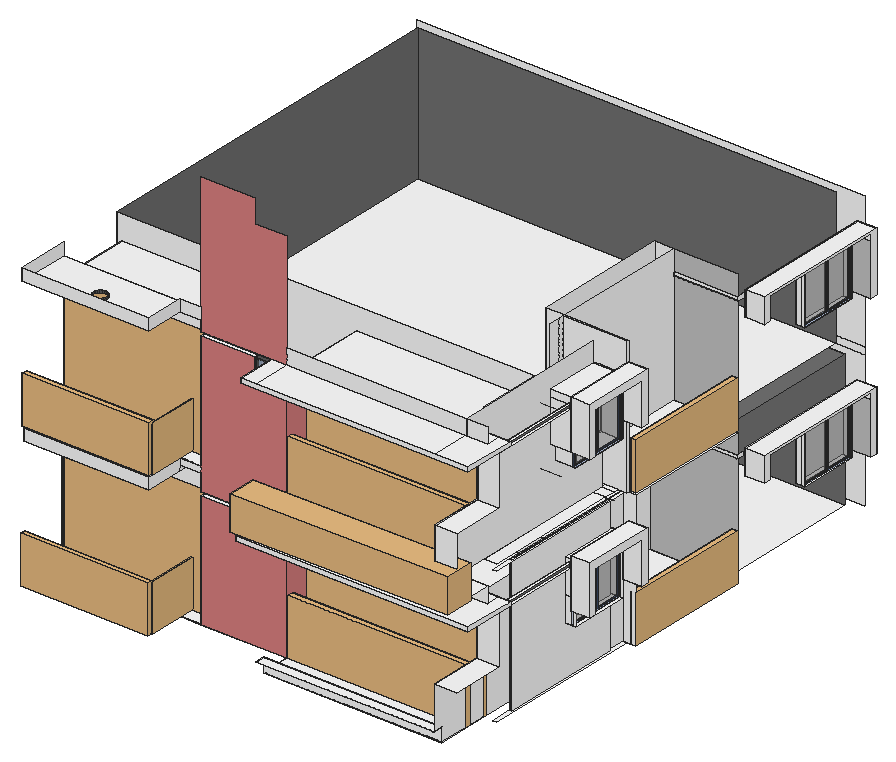
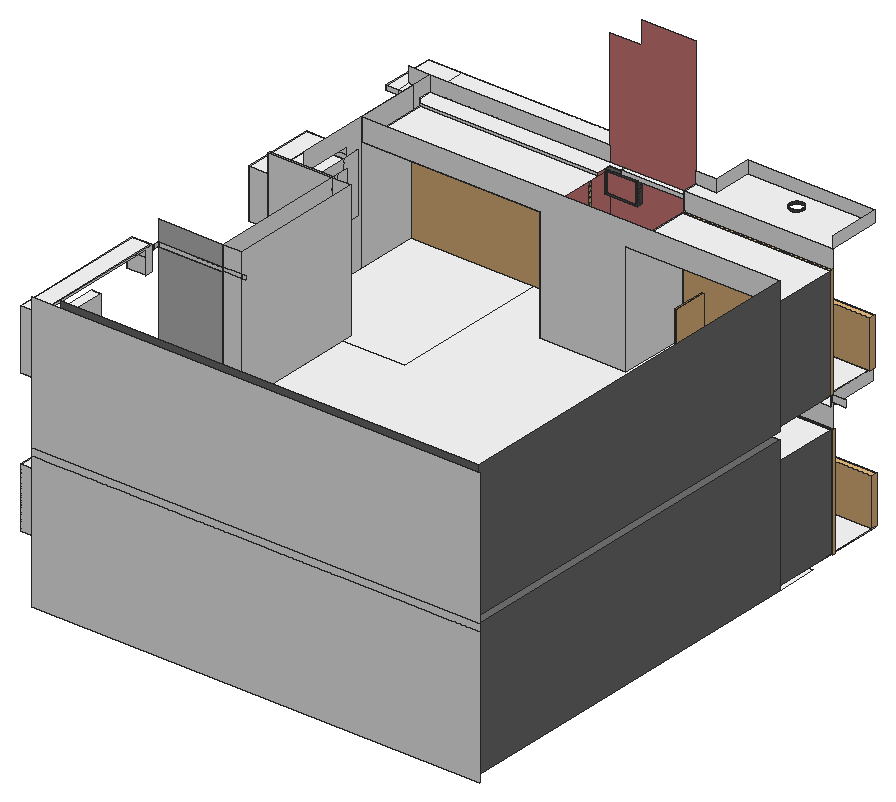
# SketchUp Ruby script. Lengths in inches.
U = 1.inch
M = Sketchup.active_model
def pt(a) = Geom::Point3d.new(a.map { |v| v * U })
def face(e, loops, mat)
  f = e.add_face(loops[0].map { |a| pt(a) })
  loops[1..].each { |l| e.add_face(l.map { |a| pt(a) }).erase! }
  f.material = f.back_material = mat if mat
  f
end
# faces: each face lists its corners as indices into pts; further lists are holes
def faces(e, pts, list, mat = nil) = list.each { |f| face(e, (f[0].is_a?(Array) ? f : [f]).map { |l| l.map { |i| pts[i] } }, mat) }
# xy, xz, yz: faces in a plane at the given z, y or x. An outline is a flat list of corners, or four numbers for a rectangle; further outlines are holes
def ring(l) = l.size == 4 ? [[l[0], l[1]], [l[2], l[1]], [l[2], l[3]], [l[0], l[3]]] : l.each_slice(2).to_a
def flat(e, list, mat, &to3) = list.each { |f| face(e, (f[0].is_a?(Array) ? f : [f]).map { |l| ring(l).map { |u, v| to3.(u, v) } }, mat) }
def xy(e, z, list, mat = nil) = flat(e, list, mat) { |x, y| [x, y, z] }
def xz(e, y, list, mat = nil) = flat(e, list, mat) { |x, z| [x, y, z] }
def yz(e, x, list, mat = nil) = flat(e, list, mat) { |y, z| [x, y, z] }
def lines(e, pts, list) = list.each { |a, b| e.add_line(pt(pts[a]), pt(pts[b])) }
# prism: a flat outline (further loops are holes) pulled along v
def prism(e, loops, v, mat = nil)
  f = face(e, loops, mat); d = Geom::Vector3d.new(v.map { |x| x * U })
  f.pushpull(f.normal.samedirection?(d) ? d.length : -d.length)
end
def box(e, o, s, mat = nil) = prism(e, [[o, [o[0] + s[0], o[1], o[2]], [o[0] + s[0], o[1] + s[1], o[2]], [o[0], o[1] + s[1], o[2]]]], [0, 0, s[2]], mat)
def at(x, y, z, deg = 0) = Geom::Transformation.translation(pt([x, y, z])) * Geom::Transformation.rotation(ORIGIN, Z_AXIS, deg.degrees)
def axes(o, x, y, z) = Geom::Transformation.new([*x, 0, *y, 0, *z, 0, *pt(o).to_a, 1])
def part(name) = M.definitions.add(name)
# library, detail: a bought-in or finely detailed component or shape, given as its bounding box
def library(name, o, s) = part(name).tap { |d| box(d.entities, o, s) }
def detail(e, o, s) = box(e.add_group.entities, o, s)
def put(e, d, t, mat = nil) = e.add_instance(d, t).tap { |i| i.material = mat if mat }
def group(e, t, mat = nil) = e.add_group.tap { |g| g.transformation = t; g.material = mat if mat }.entities
root = M.entities
M.materials.add("[Color M00]").color = [255, 255, 255]
M.materials.add("[Color M02]").color = [198, 198, 198]
M.materials.add("[Color M05]").color = [114, 114, 114]
M.materials.add("[Color M06]").color = [86, 86, 86]
M.materials.add("[Color_006]").color = [86, 86, 86]
M.materials.add("[Tile Various Tan]").color = [221, 130, 130]
M.materials.add("[Translucent Glass Blue]").color = [74, 111, 178]
M.materials["[Translucent Glass Blue]"].alpha = 0.26
M.materials.add("[Translucent Glass Gray]").color = [128, 128, 128]
M.materials["[Translucent Glass Gray]"].alpha = 0.5
M.materials.add("[Translucent_Glass_Gray]").color = [167, 187, 214]
M.materials["[Translucent_Glass_Gray]"].alpha = 0.8
c1 = library("Glazed balcony doors",[0,0,0],[135.86,2.83,115.35])
c2 = library("Glass Railing",[0,0,0],[139.5,4.76,42])
c3 = part("glass-railing")
detail(c3.entities,[0,0,0],[1.26,75.59,33.1875])
c4 = part("Group\#3")
xy(c4.entities,0,[[0,0,32.48,1.97]])
xy(c4.entities,0.98,[[0.98,0,31.5,0.98],[0.98,0.98,31.5,1.97]])
xy(c4.entities,8.86,[[0.98,0,31.5,0.98],[0.98,0.98,31.5,1.97]])
xy(c4.entities,9.84,[[0,0,32.48,1.97]])
xz(c4.entities,0,[[[0,0,32.48,9.84],[0.98,0.98,31.5,8.86]]])
xz(c4.entities,0.98,[[0.98,0.98,31.5,8.86]],"[Translucent Glass Gray]")
xz(c4.entities,1.97,[[[0,0,32.48,9.84],[0.98,0.98,31.5,8.86]]])
yz(c4.entities,0,[[0,0,1.97,9.84]])
yz(c4.entities,0.98,[[0,0.98,0.98,8.86],[0.98,0.98,1.97,8.86]])
yz(c4.entities,31.5,[[0,0.98,0.98,8.86],[0.98,0.98,1.97,8.86]])
yz(c4.entities,32.48,[[0,0,1.97,9.84]])
c5 = part("Group\#4")
xy(c5.entities,0,[[0,0,32.48,1.97]])
xy(c5.entities,0.98,[[0.98,0,31.5,0.98],[0.98,0.98,31.5,1.97]])
xy(c5.entities,71.85,[[0.98,0,31.5,0.98],[0.98,0.98,31.5,1.97]])
xy(c5.entities,72.83,[[0,0,32.48,1.97]])
xz(c5.entities,0,[[[0,0,32.48,72.83],[0.98,0.98,31.5,71.85]]])
xz(c5.entities,0.98,[[0.98,0.98,31.5,71.85]],"[Translucent Glass Gray]")
xz(c5.entities,1.97,[[[0,0,32.48,72.83],[0.98,0.98,31.5,71.85]]])
yz(c5.entities,0,[[0,0,1.97,72.83]])
yz(c5.entities,0.98,[[0,0.98,0.98,71.85],[0.98,0.98,1.97,71.85]])
yz(c5.entities,31.5,[[0,0.98,0.98,71.85],[0.98,0.98,1.97,71.85]])
yz(c5.entities,32.48,[[0,0,1.97,72.83]])
c6 = part("Fixed transom window")
xy(c6.entities,0,[[0,0,70.86,3.9375]])
xy(c6.entities,1.97,[[1.97,0,34.45,0.98],[36.42,0,68.9,3.9375],[1.97,2.95,34.45,3.9375]])
xy(c6.entities,86.61,[[1.97,0,34.45,3.9375],[34.45,0,36.42,3.9375],[36.42,0,68.9,3.9375]])
xy(c6.entities,88.58,[[0,0,70.86,3.9375]])
xz(c6.entities,0,[[[0,0,70.86,88.58],[1.97,1.97,34.45,86.61],[36.42,1.97,68.9,86.61]]])
xz(c6.entities,3.9375,[[[0,0,70.86,88.58],[1.97,1.97,34.45,86.61],[36.42,1.97,68.9,86.61]]])
yz(c6.entities,0,[[0,0,3.9375,88.58]])
yz(c6.entities,1.97,[[0,1.97,3.9375,74.8],[0,76.77,3.9375,86.61]])
yz(c6.entities,34.45,[[0,1.97,3.9375,86.61]])
yz(c6.entities,36.42,[[0,1.97,3.9375,86.61]])
yz(c6.entities,68.9,[[0,1.97,3.9375,86.61]])
yz(c6.entities,70.86,[[0,0,3.9375,88.58]])
g1 = group(c6.entities,at(1.97,0,74.8))
box(g1,[0,0,0],[66.93,3.9375,1.97])
put(c6.entities,c4,at(1.97,0.98,76.77),"[Translucent Glass Blue]")
put(c6.entities,c4,at(36.42,0.98,76.77),"[Translucent Glass Blue]")
put(c6.entities,c5,at(1.97,0.98,1.97),"[Translucent Glass Blue]")
put(c6.entities,c5,at(36.42,0.98,1.97),"[Translucent Glass Blue]")
c7 = part("FIXED+GLASS+WINDOW+WITH+TRANSOM")
put(c7.entities,c6,at(0,0,0),"[Translucent Glass Blue]")
c8 = part("BIC_Bike Shop - Window - Small")
xy(c8.entities,-8,[[[0,0,36,36],[2,2,34,34]]],"[Color_006]")
xy(c8.entities,-4,[[2,2,34,34]],"[Translucent_Glass_Gray]")
xy(c8.entities,0,[[[0,0,36,36],[2,2,34,34]]],"[Color_006]")
xz(c8.entities,0,[[0,-8,36,0]],"[Color_006]")
xz(c8.entities,2,[[2,-8,34,-4],[2,-4,34,0]],"[Color_006]")
xz(c8.entities,34,[[2,-8,34,-4],[2,-4,34,0]],"[Color_006]")
xz(c8.entities,36,[[0,-8,36,0]],"[Color_006]")
yz(c8.entities,0,[[0,-8,36,0]],"[Color_006]")
yz(c8.entities,2,[[2,-8,34,-4],[2,-4,34,0]],"[Color_006]")
yz(c8.entities,34,[[2,-8,34,-4],[2,-4,34,0]],"[Color_006]")
yz(c8.entities,36,[[0,-8,36,0]],"[Color_006]")
c9 = library("Living wall panel",[-0.54,-4.26,-5.13],[55.52,26.12,125.59])
xy(root,131.5625,[[73.74,83.25,73.74,137.58,204.98,137.58,204.98,129.875,186.35,129.875,186.35,83.25],[281.18,91.3,439.11,137.58],[186.35,117.625,204.98,129.875],[204.98,117.625,281.18,129.875],[204.98,129.875,281.18,156.83],
  [73.74,137.58,204.98,137.58,204.98,194.2,281.18,194.2,281.18,137.58,344.25,137.58,344.25,394.46,447.125,394.46,447.125,527.42,69.2,527.42,69.2,194.2,73.74,194.2],[344.25,137.58,346.4375,281.78],[346.4375,137.58,381.25,281.78],[381.25,137.58,439.11,137.58,439.11,194.2,447.125,194.2,447.125,265.65,381.25,265.65],[447.125,137.58,450.92,137.58,450.92,281.78,447.125,281.78,447.125,265.65,448.5625,265.65,448.5625,156.83,447.125,156.83],
  [69.2,156.83,73.74,194.2],[204.98,156.83,281.18,194.2],[447.125,156.83,448.5625,265.65],[381.25,265.65,447.125,281.78],[344.25,281.78,346.4375,394.46],
  [346.4375,281.78,381.25,394.46],[381.25,281.78,447.125,394.46],[447.125,281.78,450.92,394.46],[450.92,281.78,458.625,394.46]],"[Color M00]")
xy(root,131.8125,[[73.74,83.25,186.35,83.25,186.35,129.875,204.98,129.875,204.98,137.58,73.74,137.58],[281.18,91.3,439.11,137.58],[186.35,117.625,204.98,129.875]],"[Color M00]")
xy(root,143.75,[[281.18,83.25,439.11,91.3]],"[Color M00]")
xy(root,144,[[281.18,83.25,439.11,91.3]],"[Color M00]")
xy(root,175.98,[[438.17,215.57,446.875,224.27],[446.875,215.57,458.625,267.63],[438.17,224.27,446.875,267.63],[450.92,468.92,458.625,520.98]],"[Color M00]")
xy(root,181.84,[[439.11,83.25,458.625,129.875]],"[Color M00]")
xy(root,182.24,[[458.625,520.98,475.5625,526.98]],"[Color M00]")
xy(root,190.95,[[458.625,210.07,475.5625,215.57],[458.625,267.63,475.5625,273.63]],"[Color M00]")
xy(root,213.36,[[458.625,402.98,475.5625,408.98]],"[Color M00]")
xy(root,213.54,[[252.64,117.625,281.18,122.0625]],"[Tile Various Tan]")
xy(root,225.21,[[456.375,130.82,458.625,210.07]],"[Color M00]")
xy(root,228.05,[[438.17,215.57,446.875,224.27],[446.875,215.57,458.625,267.63],[458.625,215.57,475.5625,267.63],[438.17,224.27,446.875,267.63],[450.92,468.92,458.625,520.98]],"[Color M00]")
xy(root,229.21,[[456.375,130.82,458.625,210.07]],"[Color M00]")
xy(root,230.19,[[381.25,394.46,458.25,394.83]],"[Color M00]")
xy(root,230.48,[[73.74,129.875,204.98,194.2]],"[Color M00]")
xy(root,232.125,[[281.18,129.875,439.11,194.2]],"[Color M00]")
xy(root,233.48,[[381.25,394.46,458.25,394.83],[458.25,394.46,458.625,400.46]],"[Color M00]")
xy(root,233.49,[[458.625,408.98,475.5625,520.98]],"[Color M00]")
xy(root,233.52,[[263.21,83.25,263.21,122.0625,281.18,122.0625,281.18,129.875,468.99,129.875,468.99,83.25],[204.98,117.625,252.64,122.0625]],"[Color M00]")
xy(root,234.64,[[458.625,210.07,475.5625,273.63]],"[Color M00]")
xy(root,235.3,[[458.625,402.98,475.5625,526.98]],"[Color M00]")
xy(root,237.2,[[263.21,83.25,468.99,83.25,468.99,129.875,458.625,129.875,458.625,117.625,263.21,117.625],[204.98,117.625,263.21,122.0625],[439.24,117.625,458.625,129.875]],"[Color M00]")
xy(root,246.9375,[[[75.56,83.25,75.56,129.875,186.34,129.875,186.35,117.625,186.35,83.25],[129.49,93.91,131.04,94.12,132.49,94.72,133.73,95.67,134.68,96.91,135.28,98.36,135.49,99.91,135.28,101.46,134.68,102.91,133.73,104.15,132.49,105.11,131.04,105.71,129.49,105.91,127.93,105.71,126.49,105.11,125.24,104.15,124.29,102.91,123.69,101.46,123.49,99.91,123.69,98.36,124.29,96.91,125.24,95.67,126.49,94.72,127.93,94.12]]],"[Color M00]")
xy(root,248.8125,[[129.49,93.91,127.93,94.12,126.49,94.72,125.24,95.67,124.29,96.91,123.69,98.36,123.49,99.91,123.69,101.46,124.29,102.91,125.24,104.15,126.49,105.11,127.93,105.71,129.49,105.91,131.04,105.71,132.49,105.11,133.73,104.15,134.68,102.91,135.28,101.46,135.49,99.91,135.28,98.36,134.68,96.91,133.73,95.67,132.49,94.72,131.04,94.12]],"[Color M06]")
xy(root,251.5625,[[281.18,83.25,458.625,117.625],[186.35,117.625,186.34,129.875,204.98,129.875,204.98,117.625],[447.125,137.58,447.125,156.83,448.5625,156.83,448.5625,265.65,447.125,265.65,447.125,281.78,450.92,281.78,450.92,137.58],[447.125,156.83,448.5625,265.65],[344.25,194.2,346.4375,281.78],
  [346.4375,194.2,381.25,281.78],[381.25,194.2,447.125,265.65],[381.25,265.65,447.125,281.78],[344.25,281.78,346.4375,394.46],[346.4375,281.78,381.25,394.46],
  [381.25,281.78,447.125,394.46],[447.125,281.78,450.92,394.46],[450.92,281.78,458.625,394.46]],"[Color M00]")
xy(root,251.5625,[[69.2,194.2,69.2,527.42,447.125,527.42,447.125,394.46,344.25,394.46,344.25,194.2]],"[Color M05]")
xy(root,257.5625,[[75.56,83.25,75.56,129.875,73.74,129.875,73.74,137.58,204.98,137.58,204.98,117.625,186.35,117.625,186.35,83.25],[281.18,91.3,439.11,137.58],[73.74,137.58,204.98,137.58,204.98,194.2,281.18,194.2,281.18,137.58,330.6875,137.58,330.6875,281.78,385.6875,281.78,385.6875,394.46,439.42,394.46,439.42,527.42,69.2,527.42,69.2,194.2,73.74,194.2],[330.6875,137.58,439.11,137.58,439.11,194.2,439.42,194.2,439.42,257.51,401.8125,257.51,401.8125,273.63,385.6875,273.63,385.6875,281.78,330.6875,281.78],[439.42,137.58,439.8125,257.51],
  [439.8125,137.58,450.92,257.51],[401.8125,257.51,439.42,267.63],[439.42,257.51,439.8125,267.63],[439.8125,257.51,450.92,267.63],[401.8125,267.63,439.42,272.07],
  [439.42,267.63,450.92,272.07],[401.8125,272.07,439.42,273.63],[439.42,272.07,450.92,273.63],[450.92,272.07,458.625,273.63],[385.6875,273.63,401.8125,281.78],
  [401.8125,273.63,439.42,394.46],[439.42,273.63,450.92,394.46],[450.92,273.63,458.625,394.46],[385.6875,281.78,401.8125,394.46]],"[Color M00]")
xy(root,257.8125,[[75.56,83.25,186.35,83.25,186.35,117.625,204.98,117.625,204.98,137.58,73.74,137.58,73.74,129.875,75.56,129.875],[281.18,91.3,439.11,137.58]],"[Color M00]")
xy(root,271.375,[[281.18,83.25,439.11,91.3]],"[Color M00]")
xy(root,271.625,[[281.18,83.25,439.11,91.3]],"[Color M00]")
xy(root,301.98,[[439.8125,215.57,458.625,266.45],[450.92,468.92,458.625,520.98]],"[Color M00]")
xy(root,307.84,[[439.11,83.25,439.8125,129.875],[439.8125,83.25,458.625,129.875]],"[Color M00]")
xy(root,308.24,[[458.625,520.98,459,526.98],[459,520.98,475.5625,526.98]],"[Color M00]")
xy(root,316.95,[[439.8125,210.07,458.625,215.57],[458.625,210.07,475.5625,215.57],[458.625,267.63,475.5625,273.63]],"[Color M00]")
xy(root,339.36,[[458.625,402.98,459,408.98],[459,402.98,475.5625,408.98]],"[Color M00]")
xy(root,340.41,[[252.64,117.625,281.18,121.875]],"[Tile Various Tan]")
xy(root,351.21,[[456.375,130.82,458.625,210.07]],"[Color M00]")
xy(root,354.05,[[438.17,215.57,438.17,267.63,439.8125,267.63,439.8125,266.45,458.625,266.45,458.625,215.57],[458.625,215.57,475.5625,267.63],[439.8125,266.45,458.625,267.63],[450.92,468.92,458.625,520.98]],"[Color M00]")
xy(root,355.21,[[456.375,130.82,458.625,210.07]],"[Color M00]")
xy(root,356.19,[[401.8125,394.46,458.625,394.83]],"[Color M00]")
xy(root,356.48,[[73.74,129.875,204.98,194.2]],"[Color M00]")
xy(root,358.125,[[281.18,129.875,439.11,194.2]],"[Color M00]")
xy(root,359.48,[[401.8125,394.46,458.625,394.83],[458.625,394.46,459,400.46]],"[Color M00]")
xy(root,359.49,[[458.625,408.98,459,520.98],[459,408.98,475.5625,520.98]],"[Color M00]")
xy(root,360.39,[[267.36,83.25,267.36,121.875,281.18,121.875,281.18,129.875,468.99,129.875,468.99,83.25],[204.98,117.625,252.64,121.875]],"[Color M00]")
xy(root,360.64,[[439.8125,210.07,458.625,257.51],[458.625,210.07,475.5625,273.63]],"[Color M00]")
xy(root,361.3,[[458.625,402.98,459,526.98],[459,402.98,475.5625,526.98]],"[Color M00]")
xy(root,364.08,[[267.36,83.25,281.18,117.625],[281.18,83.25,439.24,117.625],[439.24,83.25,468.99,83.25,468.99,129.875,458.625,129.875,458.625,117.625,439.24,117.625],[204.98,117.625,267.36,121.875],[439.24,117.625,439.8125,129.875],
  [439.8125,117.625,458.625,129.875]],"[Color M00]")
xy(root,372.9375,[[[73.74,83.25,73.74,129.875,204.98,129.875,204.98,117.625,186.35,117.625,186.35,83.25],[129.49,93.91,131.04,94.12,132.49,94.72,133.73,95.67,134.68,96.91,135.28,98.36,135.49,99.91,135.28,101.46,134.68,102.91,133.73,104.15,132.49,105.11,131.04,105.71,129.49,105.91,127.93,105.71,126.49,105.11,125.24,104.15,124.29,102.91,123.69,101.46,123.49,99.91,123.69,98.36,124.29,96.91,125.24,95.67,126.49,94.72,127.93,94.12]]],"[Color M00]")
xz(root,83.25,[[73.74,131.5625,186.35,131.8125],[281.18,143.75,439.11,144],[263.21,233.52,468.99,237.2],[75.56,246.9375,186.35,257.5625],[281.18,251.5625,458.625,251.5625,458.625,257.5625,439.8125,257.5625,439.8125,307.84,439.11,307.84,439.11,271.375,281.18,271.375],
  [75.56,257.5625,186.35,257.8125],[439.8125,257.5625,458.625,307.84],[281.18,271.375,439.11,271.625],[267.36,360.39,468.99,364.08],[73.74,372.9375,186.35,383.5625]],"[Color M00]")
xz(root,91.3,[[281.18,131.5625,439.11,131.8125],[281.18,131.8125,439.11,143.75],[281.18,143.75,439.11,144],[281.18,257.5625,439.11,257.8125],[281.18,257.8125,439.11,271.375],
  [281.18,271.375,439.11,271.625]],"[Color M00]")
xz(root,117.625,[[186.35,131.5625,204.98,131.8125],[281.18,237.2,458.625,251.5625],[186.35,251.5625,204.98,257.5625],[186.35,257.5625,204.98,257.8125],[281.18,364.08,439.8125,377.5625],
  [439.8125,364.08,458.625,377.5625],[186.35,372.9375,204.98,383.5625]],"[Color M00]")
xz(root,117.625,[[204.98,131.5625,281.18,131.5625,281.18,213.54,252.64,213.54,252.64,233.52,204.98,233.52],[204.98,237.2,281.18,237.2,281.18,340.41,252.64,340.41,252.64,360.39,204.98,360.39],[204.98,364.08,281.18,364.08,281.18,466.54,252.64,466.54,252.64,486.52,204.98,486.52]],"[Tile Various Tan]")
xz(root,121.875,[[204.98,360.39,267.36,364.08]],"[Color M00]")
xz(root,121.875,[[252.64,340.41,281.18,360.39]],"[Tile Various Tan]")
xz(root,122.0625,[[204.98,233.52,263.21,237.2]],"[Color M00]")
xz(root,122.0625,[[252.64,213.54,281.18,233.52]],"[Tile Various Tan]")
xz(root,129.875,[[186.35,131.5625,204.98,131.8125],[439.11,181.84,458.625,181.84,458.625,233.52,281.18,233.52,281.18,232.125,439.11,232.125],[73.74,230.48,204.98,230.48,204.98,251.5625,186.34,251.5625,186.34,246.9375,75.56,246.9375,75.56,251.5625,73.74,251.5625],[439.24,233.52,458.625,237.2],[458.625,233.52,468.99,237.2],
  [61.5,251.5625,73.74,257.5625],[73.74,251.5625,75.56,257.5625],[73.74,257.5625,75.56,257.8125],[439.11,307.84,439.8125,307.84,439.8125,360.39,281.18,360.39,281.18,358.125,439.11,358.125],[439.8125,307.84,458.625,360.39],
  [73.74,356.48,204.98,372.9375],[439.24,360.39,439.8125,364.08],[439.8125,360.39,458.625,364.08],[458.625,360.39,468.99,364.08]],"[Color M00]")
xz(root,130.82,[[456.375,225.21,458.625,229.21],[456.375,351.21,458.625,355.21]],"[Color M00]")
xz(root,137.58,[[73.74,131.5625,204.98,131.8125],[281.18,131.5625,344.25,131.8125],[344.25,131.5625,346.4375,131.8125],[346.4375,131.5625,381.25,131.8125],[381.25,131.5625,439.11,131.8125],
  [73.74,257.5625,204.98,257.8125],[281.18,257.5625,330.6875,257.8125],[330.6875,257.5625,439.11,257.8125]],"[Color M00]")
xz(root,156.83,[[447.125,131.5625,448.5625,251.5625]],"[Color M00]")
xz(root,194.2,[[69.2,131.5625,69.2,251.5625,447.125,251.5625,447.125,131.5625,439.11,131.5625,439.11,232.125,281.18,232.125,281.18,131.5625,204.98,131.5625,204.98,230.48,73.74,230.48,73.74,131.5625],[69.2,257.5625,69.2,377.5625,439.42,377.5625,439.42,257.5625,439.11,257.5625,439.11,358.125,281.18,358.125,281.18,257.5625,204.98,257.5625,204.98,356.48,73.74,356.48,73.74,257.5625]],"[Color M00]")
xz(root,210.07,[[458.625,190.95,475.5625,234.64],[456.375,225.21,458.625,229.21],[439.8125,316.95,439.8125,354.05,456.375,354.05,456.375,351.21,458.625,351.21,458.625,316.95],[458.625,316.95,475.5625,360.64],[456.375,351.21,458.625,354.05],
  [439.8125,354.05,439.8125,360.64,458.625,360.64,458.625,355.21,456.375,355.21,456.375,354.05],[456.375,354.05,458.625,355.21]],"[Color M00]")
xz(root,215.57,[[438.17,175.98,446.875,228.05],[446.875,175.98,458.625,197.83],[458.625,190.95,475.5625,228.05],[446.875,197.83,458.625,228.05],[438.17,301.98,438.17,354.05,458.625,354.05,458.625,316.95,439.8125,316.95,439.8125,301.98],
  [439.8125,301.98,458.625,316.95],[458.625,316.95,475.5625,354.05]],"[Color M00]")
xz(root,224.27,[[438.17,175.98,446.875,228.05]],"[Color M00]")
xz(root,265.65,[[381.25,131.5625,447.125,251.5625],[447.125,131.5625,448.5625,251.5625]],"[Color M00]")
xz(root,266.45,[[439.8125,301.98,458.625,354.05]],"[Color M00]")
xz(root,267.63,[[438.17,175.98,446.875,228.05],[446.875,175.98,458.625,228.05],[458.625,190.95,475.5625,228.05],[438.17,301.98,439.8125,354.05],[439.8125,301.98,458.625,316.95],
  [439.8125,316.95,458.625,354.05],[458.625,316.95,475.5625,354.05]],"[Color M00]")
xz(root,272.07,[[401.8125,257.5625,458.625,377.5625]],"[Color M00]")
xz(root,273.63,[[458.625,190.95,475.5625,234.64],[385.6875,257.5625,401.8125,377.5625],[401.8125,257.5625,458.625,377.5625],[458.625,316.95,475.5625,360.64]],"[Color M00]")
xz(root,281.78,[[344.25,131.5625,346.4375,251.5625],[346.4375,131.5625,381.25,251.5625],[381.25,131.5625,447.125,251.5625],[447.125,131.5625,458.625,251.5625]],"[Color M00]")
xz(root,394.46,[[344.25,131.5625,346.4375,251.5625],[346.4375,131.5625,381.25,251.5625],[385.6875,257.5625,401.8125,356.19],[381.625,356.19,385.6875,359.48],[385.6875,356.19,401.8125,359.48],
  [385.6875,359.48,401.8125,377.5625]],"[Color M00]")
xz(root,394.46,[[381.25,131.5625,458.625,230.19],[381.25,233.48,458.625,251.5625],[401.8125,257.5625,458.625,356.19],[401.8125,359.48,458.625,377.5625]],"[Color M02]")
xz(root,394.83,[[381.25,230.19,458.25,233.48],[401.8125,356.19,458.625,359.48]],"[Color M00]")
xz(root,400.46,[[458.25,230.11,458.625,233.48],[458.625,356.11,459,359.48]],"[Color M00]")
xz(root,402.98,[[458.625,213.36,475.5625,235.3],[458.625,339.36,459,361.3],[459,339.36,475.5625,361.3]],"[Color M00]")
xz(root,408.98,[[458.625,213.36,475.5625,227.49],[458.625,227.49,475.5625,233.49],[458.625,339.36,459,353.49],[459,339.36,475.5625,353.49],[458.625,353.49,459,359.49],
  [459,353.49,475.5625,359.49]],"[Color M00]")
xz(root,468.92,[[450.92,175.98,458.625,228.05],[450.92,301.98,458.625,354.05]],"[Color M00]")
xz(root,520.98,[[450.92,175.98,458.625,228.05],[458.625,228.05,475.5625,233.49],[450.92,301.98,458.625,354.05],[458.625,308.24,459,354.05],[458.625,354.05,459,359.49],
  [459,354.05,475.5625,359.49]],"[Color M00]")
xz(root,520.98,[[458.625,182.24,475.5625,228.05],[459,308.24,475.5625,354.05]],"[Color M02]")
xz(root,526.98,[[458.625,182.24,475.5625,235.3],[458.625,308.24,459,361.3],[459,308.24,475.5625,361.3]],"[Color M00]")
xz(root,527.42,[[69.2,131.5625,447.125,251.5625],[69.2,257.5625,439.42,377.5625]],"[Color M05]")
xz(root,535.125,[[61.5,131.5625,458.625,251.5625],[61.5,251.5625,458.625,257.5625],[61.5,257.5625,458.625,377.5625]],"[Color M00]")
yz(root,69.2,[[194.2,131.5625,527.42,251.5625],[194.2,257.5625,527.42,377.5625]],"[Color M05]")
yz(root,73.74,[[83.25,131.5625,129.875,131.8125],[129.875,131.5625,137.58,131.8125],[129.875,257.5625,137.58,257.8125],[83.25,372.9375,129.875,383.5625]],"[Color M00]")
yz(root,73.74,[[137.58,131.5625,194.2,131.5625,194.2,230.48,129.875,230.48,129.875,131.8125,137.58,131.8125],[137.58,257.5625,194.2,257.5625,194.2,356.48,129.875,356.48,129.875,257.8125,137.58,257.8125]],"[Color M05]")
yz(root,75.56,[[83.25,246.9375,129.875,257.5625],[83.25,257.5625,129.875,257.8125]],"[Color M00]")
yz(root,186.35,[[83.25,131.5625,117.625,131.8125],[117.625,131.5625,129.875,131.8125],[83.25,246.9375,117.625,257.5625],[83.25,257.5625,117.625,257.8125],[83.25,372.9375,117.625,383.5625]],"[Color M00]")
yz(root,204.98,[[117.625,131.5625,129.875,131.8125],[137.58,131.5625,137.58,131.8125,117.625,131.8125,117.625,230.48,194.2,230.48,194.2,131.5625],[129.875,131.5625,137.58,131.8125],[117.625,230.48,117.625,233.52,122.0625,233.52,122.0625,237.2,117.625,237.2,117.625,251.5625,129.875,251.5625,129.875,230.48],[117.625,257.5625,137.58,257.8125],
  [137.58,257.5625,137.58,257.8125,117.625,257.8125,117.625,356.48,194.2,356.48,194.2,257.5625],[117.625,356.48,117.625,360.39,121.875,360.39,121.875,364.08,117.625,364.08,117.625,372.9375,129.875,372.9375,129.875,356.48]],"[Color M00]")
yz(root,252.64,[[117.625,213.54,122.0625,233.52],[117.625,340.41,121.875,360.39]],"[Tile Various Tan]")
yz(root,263.21,[[83.25,233.52,122.0625,237.2]],"[Color M00]")
yz(root,267.36,[[83.25,360.39,121.875,364.08]],"[Color M00]")
yz(root,281.18,[[91.3,131.5625,117.625,131.8125],[117.625,131.5625,129.875,131.8125],[129.875,131.5625,137.58,131.8125],[83.25,143.75,91.3,144],[83.25,251.5625,83.25,271.375,91.3,271.375,91.3,257.5625,117.625,257.5625,117.625,251.5625],
  [91.3,257.5625,117.625,257.8125],[117.625,257.5625,137.58,257.8125],[83.25,271.375,91.3,271.625]],"[Color M00]")
yz(root,281.18,[[137.58,131.5625,194.2,131.5625,194.2,232.125,122.0625,232.125,122.0625,213.54,117.625,213.54,117.625,131.8125,137.58,131.8125],[122.0625,232.125,129.875,233.52],[137.58,257.5625,194.2,257.5625,194.2,358.125,121.875,358.125,121.875,340.41,117.625,340.41,117.625,257.8125,137.58,257.8125],[121.875,358.125,129.875,360.39]],"[Tile Various Tan]")
yz(root,344.25,[[281.78,131.5625,394.46,251.5625]],"[Color M00]")
yz(root,346.4375,[[281.78,131.5625,394.46,251.5625]],"[Color M00]")
yz(root,381.25,[[265.65,131.5625,281.78,251.5625],[281.78,131.5625,394.46,251.5625],[394.46,230.19,394.83,233.48]],"[Color M00]")
yz(root,385.6875,[[273.63,257.5625,394.46,377.5625]],"[Color M00]")
yz(root,401.8125,[[257.51,257.5625,267.63,377.5625],[267.63,257.5625,272.07,377.5625],[272.07,257.5625,273.63,377.5625],[273.63,257.5625,394.46,377.5625],[394.46,356.19,394.83,359.48]],"[Color M00]")
yz(root,438.17,[[215.57,175.98,224.27,228.05],[224.27,175.98,267.63,228.05],[199.45,301.98,215.57,354.05],[215.57,301.98,267.63,354.05]],"[Color M00]")
yz(root,439.11,[[137.58,131.5625,137.58,131.8125,91.3,131.8125,91.3,144,83.25,144,83.25,181.84,129.875,181.84,129.875,232.125,194.2,232.125,194.2,131.5625],[91.3,131.5625,137.58,131.8125],[83.25,143.75,91.3,144],[137.58,257.5625,137.58,257.8125,91.3,257.8125,91.3,271.625,83.25,271.625,83.25,307.84,129.875,307.84,129.875,358.125,194.2,358.125,194.2,257.5625],[91.3,257.5625,137.58,257.8125],
  [83.25,271.375,91.3,271.625]],"[Color M00]")
yz(root,439.42,[[137.58,257.5625,194.2,377.5625]],"[Color M00]")
yz(root,439.8125,[[83.25,257.5625,83.25,307.84,129.875,307.84,129.875,364.08,117.625,364.08,117.625,377.5625,257.51,377.5625,257.51,360.64,210.07,360.64,210.07,316.95,215.57,316.95,215.57,301.98,266.45,301.98,266.45,354.05,267.63,354.05,267.63,257.5625]],"[Color M00]")
yz(root,446.875,[[215.57,175.98,224.27,197.83],[224.27,175.98,267.63,228.05],[215.57,197.83,224.27,228.05]],"[Color M00]")
yz(root,447.125,[[156.83,131.5625,194.2,251.5625],[194.2,131.5625,265.65,251.5625],[265.65,131.5625,281.78,251.5625]],"[Color M00]")
yz(root,448.5625,[[156.83,131.5625,265.65,251.5625]],"[Color M00]")
yz(root,450.92,[[468.92,175.98,520.98,228.05],[468.92,301.98,520.98,354.05]],"[Color M00]")
yz(root,456.375,[[130.82,225.21,210.07,229.21],[130.82,351.21,210.07,355.21]],"[Color M05]")
yz(root,458.25,[[400.46,230.11,400.46,233.48,394.83,233.48,394.83,230.19,394.46,230.19]],"[Color M00]")
yz(root,458.625,[[520.98,182.24,520.98,233.49,408.98,233.49,408.98,213.36,402.98,213.36,402.98,235.3,526.98,235.3,526.98,182.24],[210.07,190.95,210.07,234.64,273.63,234.64,273.63,190.95,267.63,190.95,267.63,228.05,215.57,228.05,215.57,190.95],[272.07,257.5625,273.63,316.95],[520.98,308.24,520.98,359.49,408.98,359.49,408.98,339.36,402.98,339.36,402.98,361.3,526.98,361.3,526.98,308.24],[210.07,316.95,215.57,354.05],
  [267.63,316.95,272.07,360.64],[272.07,316.95,273.63,360.64],[210.07,354.05,257.51,360.64],[257.51,354.05,267.63,360.64],[394.46,356.19,394.83,359.48],
  [272.07,360.64,273.63,377.5625]],"[Color M00]")
yz(root,459,[[520.98,308.24,520.98,359.49,408.98,359.49,408.98,339.36,402.98,339.36,402.98,361.3,526.98,361.3,526.98,308.24],[400.46,356.11,400.46,359.48,394.46,359.48,394.46,356.19]],"[Color M00]")
yz(root,468.99,[[83.25,233.52,129.875,237.2],[83.25,360.39,129.875,364.08]],"[Color M00]")
yz(root,475.5625,[[520.98,182.24,526.98,182.24,526.98,235.3,402.98,235.3,402.98,213.36,408.98,213.36,408.98,233.49,520.98,233.49],[210.07,190.95,215.57,190.95,215.57,228.05,267.63,228.05,267.63,190.95,273.63,190.95,273.63,234.64,210.07,234.64],[520.98,308.24,526.98,308.24,526.98,361.3,402.98,361.3,402.98,339.36,408.98,339.36,408.98,359.49,520.98,359.49],[210.07,316.95,215.57,316.95,215.57,354.05,267.63,354.05,267.63,316.95,273.63,316.95,273.63,360.64,210.07,360.64]],"[Color M00]")
p = [[458.625,394.46,230.19],[458.625,400.46,230.11],[458.25,400.46,230.11],[458.25,394.46,230.19],[129.49,93.91,246.9375],[127.93,94.12,246.9375],
  [127.93,94.12,248.8125],[129.49,93.91,248.8125],[131.04,94.12,246.9375],[131.04,94.12,248.8125],[126.49,94.72,246.9375],[126.49,94.72,248.8125],
  [132.49,94.72,246.9375],[132.49,94.72,248.8125],[125.24,95.67,246.9375],[125.24,95.67,248.8125],[133.73,95.67,246.9375],[133.73,95.67,248.8125],
  [124.29,96.91,246.9375],[124.29,96.91,248.8125],[134.68,96.91,246.9375],[134.68,96.91,248.8125],[123.69,98.36,246.9375],[123.69,98.36,248.8125],
  [135.28,98.36,246.9375],[135.28,98.36,248.8125],[123.49,99.91,246.9375],[123.49,99.91,248.8125],[135.49,99.91,246.9375],[135.49,99.91,248.8125],
  [123.69,101.46,246.9375],[123.69,101.46,248.8125],[135.28,101.46,246.9375],[135.28,101.46,248.8125],[124.29,102.91,246.9375],[124.29,102.91,248.8125],
  [134.68,102.91,246.9375],[134.68,102.91,248.8125],[125.24,104.15,246.9375],[125.24,104.15,248.8125],[133.73,104.15,246.9375],[133.73,104.15,248.8125],
  [126.49,105.11,246.9375],[126.49,105.11,248.8125],[132.49,105.11,246.9375],[132.49,105.11,248.8125],[127.93,105.71,246.9375],[127.93,105.71,248.8125],
  [131.04,105.71,246.9375],[131.04,105.71,248.8125],[129.49,105.91,246.9375],[129.49,105.91,248.8125],[186.34,129.875,251.5625],[186.35,117.625,251.5625],
  [186.35,117.625,246.9375],[186.34,129.875,246.9375],[459,400.46,356.11],[459,394.46,356.19],[458.625,394.46,356.19],[458.625,400.46,356.11],
  [129.49,93.91,372.9375],[127.93,94.12,372.9375],[127.93,94.12,374.8125],[129.49,93.91,374.8125],[131.04,94.12,372.9375],[131.04,94.12,374.8125],
  [126.49,94.72,372.9375],[126.49,94.72,374.8125],[132.49,94.72,372.9375],[132.49,94.72,374.8125],[125.24,95.67,372.9375],[125.24,95.67,374.8125],
  [133.73,95.67,372.9375],[133.73,95.67,374.8125],[124.29,96.91,372.9375],[124.29,96.91,374.8125],[134.68,96.91,372.9375],[134.68,96.91,374.8125],
  [123.69,98.36,372.9375],[123.69,98.36,374.8125],[135.28,98.36,372.9375],[135.28,98.36,374.8125],[123.49,99.91,372.9375],[123.49,99.91,374.8125],
  [135.49,99.91,372.9375],[135.49,99.91,374.8125],[123.69,101.46,372.9375],[123.69,101.46,374.8125],[135.28,101.46,372.9375],[135.28,101.46,374.8125],
  [124.29,102.91,372.9375],[124.29,102.91,374.8125],[134.68,102.91,372.9375],[134.68,102.91,374.8125],[125.24,104.15,372.9375],[125.24,104.15,374.8125],
  [133.73,104.15,372.9375],[133.73,104.15,374.8125],[126.49,105.11,372.9375],[126.49,105.11,374.8125],[132.49,105.11,372.9375],[132.49,105.11,374.8125],
  [127.93,105.71,372.9375],[127.93,105.71,374.8125],[131.04,105.71,372.9375],[131.04,105.71,374.8125],[129.49,105.91,372.9375],[129.49,105.91,374.8125],
  [458.625,199.45,301.98],[438.17,199.45,301.98],[458.625,199.45,354.05],[438.17,199.45,354.05],[438.17,267.63,354.05],[422.05,267.63,354.05],
  [422.05,267.63,301.98],[438.17,267.63,301.98],[458.625,257.51,257.5625],[450.92,257.51,257.5625]]
faces(root,p,[[0,1,2,3],[52,53,54,55],[56,57,58,59]],"[Color M00]")
faces(root,p,[[4,5,6,7],[8,4,7,9],[5,10,11,6],[12,8,9,13],[10,14,15,11],[16,12,13,17],[14,18,19,15],[20,16,17,21],
  [18,22,23,19],[24,20,21,25],[22,26,27,23],[28,24,25,29],[26,30,31,27],[32,28,29,33],[30,34,35,31],[36,32,33,37],
  [34,38,39,35],[40,36,37,41],[38,42,43,39],[44,40,41,45],[42,46,47,43],[48,44,45,49],[46,50,51,47],[50,48,49,51],
  [60,61,62,63],[64,60,63,65],[61,66,67,62],[68,64,65,69],[66,70,71,67],[72,68,69,73],[70,74,75,71],[76,72,73,77],
  [74,78,79,75],[80,76,77,81],[78,82,83,79],[84,80,81,85],[82,86,87,83],[88,84,85,89],[86,90,91,87],[92,88,89,93],
  [90,94,95,91],[96,92,93,97],[94,98,99,95],[100,96,97,101],[98,102,103,99],[104,100,101,105],[102,106,107,103],[106,104,105,107]],"[Color M06]")
lines(root,p,[[108,109],[110,111],[112,113],[114,113],[115,114],[116,117]])
put(root,c1,axes([71.625,129.49,131.55],[0.96594,0,0],[0,0.86,0],[0,0,0.86]),"[Color M00]")
put(root,c2,axes([458.625,281.78,131.5625],[0,0.80723,0],[-1,0,0],[0,0,1]),"[Color M00]")
put(root,c2,axes([73.74,81.24,131.8125],[0.80723,0,0],[0,1,0],[0,0,1]),"[Color M00]")
put(root,c2,axes([281.18,117.625,131.8125],[1.13217,0,0],[0,1,0],[0,0,1.19122]),"[Color M00]")
put(root,c1,axes([281.18,137.58,131.8125],[1.16249,0,0],[0,0.86,0],[0,0,0.86]),"[Translucent Glass Blue]")
put(root,c3,axes([186.35,85.95,132.16],[1,0,0],[0,1,0],[0,0,1.24195]),"[Color M00]")
put(root,c7,axes([458.625,469.08,175.98],[0,0.73244,0],[-0.59,0,0],[0,0,0.57689]),"[Color M00]")
put(root,c7,axes([457.01,215.57,175.98],[0,0.73468,0],[-0.59,0,0],[0,0,0.59]),"[Color M00]")
put(root,c8,axes([252.64,117.625,213.54],[0.79273,0,0],[0,0,0.56],[0,-0.56,0]))
put(root,c9,axes([275.83,74.53,277.66],[0.0058,0,-0.53997],[0,1,0],[1.53606,0,0.0165]),"[Color M00]")
put(root,c1,axes([73.4375,129.49,257.55],[0.96594,0,0],[0,0.86,0],[0,0,0.86]),"[Color M05]")
put(root,c1,axes([281.18,137.58,257.8125],[1.16249,0,0],[0,0.86,0],[0,0,0.86]),"[Color M00]")
put(root,c2,axes([281.18,117.625,257.8125],[1.13217,0,0],[0,1,0],[0,0,1.19122]),"[Color M00]")
put(root,c3,axes([186.35,85.95,257.9],[1,0,0],[0,1,0],[0,0,1.24195]),"[Color M00]")
put(root,c2,axes([73.74,83.25,258.0625],[0.80723,0,0],[0,1,0],[0,0,1]),"[Color M00]")
put(root,c2,axes([466.38,272.07,259.99],[0,0.80723,0],[-1,0,0],[0,0,1]),"[Color M00]")
put(root,c7,axes([458.625,469.08,301.98],[0,0.73244,0],[-0.59,0,0],[0,0,0.57689]),"[Color M00]")
put(root,c7,axes([458.625,214.38,301.98],[0,0.73468,0],[-0.59,0,0],[0,0,0.59]),"[Color M00]")
put(root,c8,axes([252.64,117.625,340.41],[0.79273,0,0],[0,0,0.56],[0,-0.56,0]))
